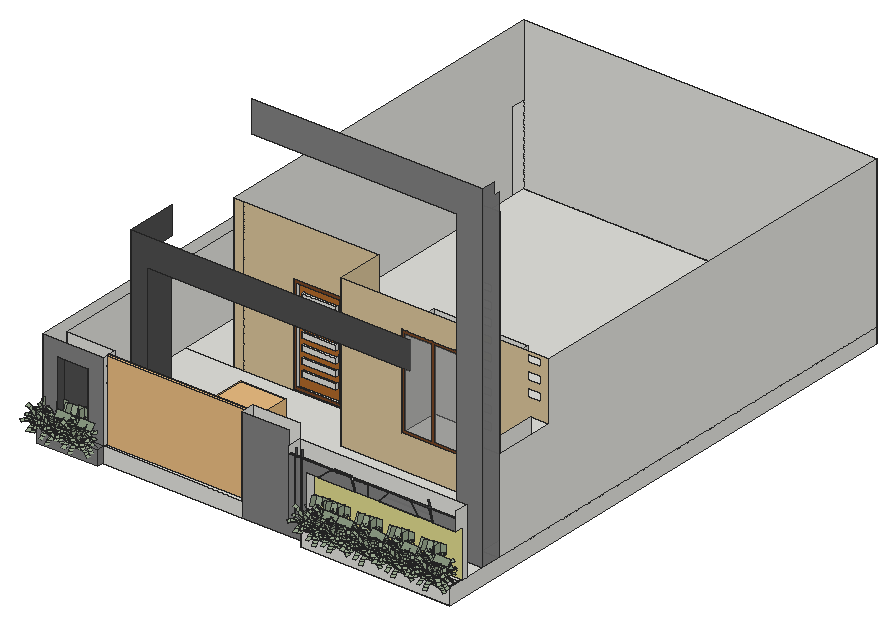
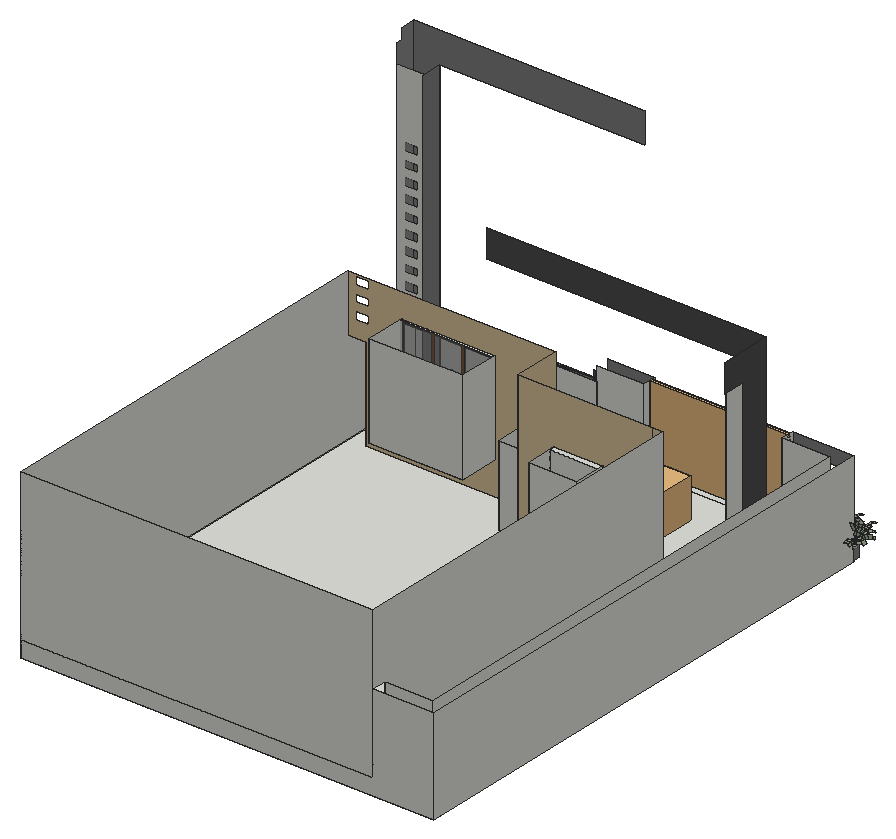
# SketchUp Ruby script. Lengths in inches.
U = 1.inch
M = Sketchup.active_model
def pt(a) = Geom::Point3d.new(a.map { |v| v * U })
def face(e, loops, mat)
  f = e.add_face(loops[0].map { |a| pt(a) })
  loops[1..].each { |l| e.add_face(l.map { |a| pt(a) }).erase! }
  f.material = f.back_material = mat if mat
  f
end
# faces: each face lists its corners as indices into pts; further lists are holes
def faces(e, pts, list, mat = nil) = list.each { |f| face(e, (f[0].is_a?(Array) ? f : [f]).map { |l| l.map { |i| pts[i] } }, mat) }
# xy, xz, yz: faces in a plane at the given z, y or x. An outline is a flat list of corners, or four numbers for a rectangle; further outlines are holes
def ring(l) = l.size == 4 ? [[l[0], l[1]], [l[2], l[1]], [l[2], l[3]], [l[0], l[3]]] : l.each_slice(2).to_a
def flat(e, list, mat, &to3) = list.each { |f| face(e, (f[0].is_a?(Array) ? f : [f]).map { |l| ring(l).map { |u, v| to3.(u, v) } }, mat) }
def xy(e, z, list, mat = nil) = flat(e, list, mat) { |x, y| [x, y, z] }
def xz(e, y, list, mat = nil) = flat(e, list, mat) { |x, z| [x, y, z] }
def yz(e, x, list, mat = nil) = flat(e, list, mat) { |y, z| [x, y, z] }
def lines(e, pts, list) = list.each { |a, b| e.add_line(pt(pts[a]), pt(pts[b])) }
# prism: a flat outline (further loops are holes) pulled along v
def prism(e, loops, v, mat = nil)
  f = face(e, loops, mat); d = Geom::Vector3d.new(v.map { |x| x * U })
  f.pushpull(f.normal.samedirection?(d) ? d.length : -d.length)
end
def box(e, o, s, mat = nil) = prism(e, [[o, [o[0] + s[0], o[1], o[2]], [o[0] + s[0], o[1] + s[1], o[2]], [o[0], o[1] + s[1], o[2]]]], [0, 0, s[2]], mat)
def at(x, y, z, deg = 0) = Geom::Transformation.translation(pt([x, y, z])) * Geom::Transformation.rotation(ORIGIN, Z_AXIS, deg.degrees)
def axes(o, x, y, z) = Geom::Transformation.new([*x, 0, *y, 0, *z, 0, *pt(o).to_a, 1])
def part(name) = M.definitions.add(name)
# library, detail: a bought-in or finely detailed component or shape, given as its bounding box
def library(name, o, s) = part(name).tap { |d| box(d.entities, o, s) }
def detail(e, o, s) = box(e.add_group.entities, o, s)
def put(e, d, t, mat = nil) = e.add_instance(d, t).tap { |i| i.material = mat if mat }
def group(e, t, mat = nil) = e.add_group.tap { |g| g.transformation = t; g.material = mat if mat }.entities
root = M.entities
M.materials.add("Generic").color = [129, 129, 129]
M.materials["Generic"].alpha = 0.97
M.materials.add("Generic\#1").color = [79, 79, 79]
M.materials.add("Generic\#3").color = [219, 197, 155]
M.materials.add("Generic\#5").color = [224, 219, 143]
M.materials.add("Generic\#6").color = [129, 129, 129]
M.materials.add("[Translucent Glass Gray]").color = [128, 128, 128]
M.materials["[Translucent Glass Gray]"].alpha = 0.28
M.materials.add("[Wood Bamboo]").color = [177, 105, 43]
M.materials.add("[Wood Board Cork]").color = [198, 185, 106]
M.materials.add("[Wood Veneer 01]").color = [120, 70, 37]
M.materials.add("hymenocallis littoralis").color = [156, 172, 146]
c1 = library("Group3\#1",[-238.15,54.18,0],[46.4,43.96,56.68])
c2 = part("Group\#856")
xy(c2.entities,7.38,[[0,0,5.5,15.91]],"hymenocallis littoralis")
p = [[5.5,28.78,0],[5.5,26.79,3.44],[0,26.79,3.44],[0,28.78,0],[0,23.75,6],[5.5,23.75,6],
  [0,15.91,7.38],[5.5,15.91,7.38]]
faces(c2.entities,p,[[0,1,2,3],[4,2,1,5],[6,4,5,7]],"hymenocallis littoralis")
c3 = part("Group\#854")
xy(c3.entities,7.38,[[0,0,5.5,15.91],[0,15.91,5.5,23.87]],"hymenocallis littoralis")
p = [[5.5,31.07,4.3],[5.5,27.74,6.47],[0,27.74,6.47],[0,31.07,4.3],[0,23.87,7.38],[5.5,23.87,7.38]]
faces(c3.entities,p,[[0,1,2,3],[4,2,1,5]],"hymenocallis littoralis")
c4 = part("Group\#857")
xy(c4.entities,7.38,[[0,0,5.6,15.91]],"hymenocallis littoralis")
p = [[5.6,28.78,0],[5.6,26.79,3.44],[0,26.79,3.44],[0,28.78,0],[0,23.75,6],[5.6,23.75,6],
  [0,15.91,7.38],[5.6,15.91,7.38]]
faces(c4.entities,p,[[0,1,2,3],[4,2,1,5],[6,4,5,7]],"hymenocallis littoralis")
c5 = part("Group\#855")
put(c5.entities,c3,axes([6.09,8.57,-0.52],[0.446,0.85617,0.26089],[-0.18444,-0.19731,0.96283],[0.87582,-0.47754,0.0699]))
put(c5.entities,c3,axes([6.29,7.28,-1.71],[0.37058,0.92707,-0.05667],[-0.32382,0.19004,0.99128],[0.87712,-0.32925,0.34964]))
put(c5.entities,c3,axes([11.04,16.14,-0.7],[1,0,0],[0,0.16628,1.02662],[0,-1.18456,0.19186]))
c6 = part("Group\#860")
put(c6.entities,c2,axes([24.57,32.05,-1.76],[0.9552,-0.22102,-0.19681],[0.4036,0.95545,0.88585],[-0.00568,-0.67859,0.7345]))
put(c6.entities,c2,axes([23.95,29.24,-2.4],[0,1,0],[-0.76041,0,0.64945],[0.64945,0,0.76041]))
put(c6.entities,c2,axes([24.22,24.72,-0.48],[-0.70711,0.70711,0],[-0.32757,-0.32757,0.80237],[0.61237,0.61237,0.5]))
put(c6.entities,c3,axes([20.66,37.22,-0.63],[1.12361,0.03262,0.39091],[-0.43499,0.29739,0.78777],[0.09852,-1.27434,0.37535]))
put(c6.entities,c2,axes([28.75,24.45,-2.4],[-1,0,0],[0,-0.76041,0.64945],[0,0.64945,0.76041]))
put(c6.entities,c4,axes([30.4,30.98,-3.7],[0.65676,-0.72002,0.22414],[0.55667,0.66341,0.5],[-0.50871,-0.20361,0.83652]))
put(c6.entities,c4,axes([32.41,29.61,-3.7],[0.04029,-0.97372,0.22414],[0.85287,0.15038,0.5],[-0.52057,0.17102,0.83652]))
put(c6.entities,c2,axes([31.89,25.85,-1.76],[-0.92056,0.33739,-0.19681],[-0.5186,-0.89824,0.88585],[0.08952,0.67268,0.7345]))
put(c6.entities,c2,axes([25.55,34.78,-0.48],[0.86603,0.5,0],[-0.25,0.43301,0.86603],[0.43301,-0.75,0.5]))
put(c6.entities,c4,axes([20.4,16.9375,-8.07],[-0.70711,0.70711,0],[-0.35754,-0.35754,0.65422],[1.3987,1.3987,1.52882]))
put(c6.entities,c2,axes([32.86,34.14,-0.48],[0.76604,-0.64279,0],[0.32139,0.38302,0.86603],[-0.55667,-0.66341,0.5]))
put(c6.entities,c2,axes([27.15,34.7,-0.1],[0.82472,-0.17528,-0.53769],[0.53769,0.53769,0.64945],[0.17528,-0.82472,0.53769]))
put(c6.entities,c2,axes([33.58,28.77,-2.4],[0,-1,0],[0.76041,0,0.64945],[-0.64945,0,0.76041]))
put(c6.entities,c2,axes([26.43,23.87,-2.81],[-0.75126,0.04415,0.65853],[0.53769,-0.53769,0.64945],[0.38276,0.84199,0.3802]))
put(c6.entities,c2,axes([28.78,23.98,-2.4],[-1,0,0],[0,-0.76041,0.64945],[0,0.64945,0.76041]))
put(c6.entities,c2,axes([25.39,25.38,-2.4],[-0.70711,0.70711,0],[-0.53769,-0.53769,0.64945],[0.45923,0.45923,0.76041]))
put(c6.entities,c2,axes([27.32,21.63,-0.1],[-0.45923,0.70711,-0.53769],[-0.76041,0,0.64945],[0.45923,0.70711,0.53769]))
put(c6.entities,c2,axes([25.17,27.625,-1.76],[0.56416,0.80187,-0.19681],[-0.66673,0.66673,0.80532],[0.62659,-0.26057,0.7345]))
put(c6.entities,c4,axes([27.59,27.04,-3.96],[-0.8993,-0.06127,0.43301],[0.2962,-0.8138,0.5],[0.32175,0.57791,0.75]))
put(c6.entities,c4,axes([26.98,24.5,-3.18],[-0.5,0.86603,0],[-0.75,-0.43301,0.5],[0.43301,0.25,0.86603]))
put(c6.entities,c4,axes([24.55,27.74,-3.7],[0.29517,0.92878,0.22414],[-0.85287,0.15038,0.5],[0.43068,-0.33875,0.83652]))
put(c6.entities,c4,axes([24.26,29.8,-3.18],[0.76604,0.64279,0],[-0.47317,0.5639,0.425],[0.32139,-0.38302,0.86603]))
put(c6.entities,c4,axes([25.98,32.46,-3.18],[1,0,0],[0,0.86603,0.5],[0,-0.5,0.86603]))
put(c6.entities,c2,axes([28.78,33.57,-2.4],[1,0,0],[0,0.76041,0.64945],[0,-0.64945,0.76041]))
put(c6.entities,c5,at(14.99,21.38,2.5))
put(c6.entities,c3,axes([34.63,26.34,-1.46],[-0.70089,-0.70877,0.07994],[0.4756,-0.38088,0.79293],[-0.53156,0.59378,0.60405]))
put(c6.entities,c3,axes([28.14,16.92,1.8125],[-1.19719,0.6912,0],[-0.09607,-0.16641,0.94244],[0.68444,1.18549,0.17613]))
put(c6.entities,c3,axes([31.5625,35.84,0.97],[0.66765,-1.1564,0.35779],[0.04445,0.30732,0.91033],[-1.20828,-0.64496,0.17012]))
put(c6.entities,c3,axes([38.94,22.51,0.89],[-0.97932,-0.67164,-0.05202],[0.27787,-0.41401,0.90999],[-0.85985,0.93577,0.32097]))
put(c6.entities,c3,axes([38.44,21.09,1.98],[-1.02864,-0.54856,0.2395],[0.33481,0.06999,0.88388],[-0.77261,1.08328,0.06417]))
put(c6.entities,c4,axes([35.02,30.51,-1.3],[-0.17365,-0.98481,0],[0.60224,-0.10619,0.79122],[-0.7792,0.13739,0.61153]))
put(c6.entities,c4,axes([29.41,22.33,-1.3],[-0.93969,0.34202,0],[-0.20915,-0.57465,0.79122],[0.27061,0.74351,0.61153]))
put(c6.entities,c3,axes([19.64,36,-1.62],[1.18194,0.09546,0.08234],[-0.14377,0.68823,0.76313],[0.21457,-1.1326,0.62386]))
put(c6.entities,c4,axes([24.25,24.14,-1.3],[-0.34202,0.93969,0],[-0.57465,-0.20915,0.79122],[0.74351,0.27061,0.61153]))
put(c6.entities,c4,axes([25.98,34.61,-1.3],[1,0,0],[0,0.61153,0.79122],[0,-0.79122,0.61153]))
put(c6.entities,c4,axes([31.16,34.41,-1.64],[0.56518,-0.80224,-0.19234],[0.73413,0.34233,0.72935],[-0.47639,-0.50772,0.71782]))
put(c6.entities,c4,axes([40.52,26.84,-5.82],[-0.42262,-0.90631,0],[0.48019,-0.22391,0.68552],[-1.43418,0.66877,1.22305]))
put(c6.entities,c2,axes([29.86,38.42,-1.01],[0.89064,-0.37013,0.26413],[-0.03924,0.63286,1.01918],[-0.45353,-0.76487,0.45748]))
put(c6.entities,c2,axes([29.34,22.4,-0.48],[-0.99619,-0.08716,0],[0.04358,-0.4981,0.86603],[-0.07548,0.86273,0.5]))
c7 = part("Group\#858")
xz(c7.entities,10.07,[[9.07,0,10.07,31.01],[0,31.01,0,45.12,20.13,45.12,20.13,31.01,10.07,31.01,10.07,32.58,9.07,32.58,9.07,31.01]],"hymenocallis littoralis")
yz(c7.entities,10.07,[[0,31.01,20.13,45.12]],"hymenocallis littoralis")
p = [[9.57,9.2,0],[10.07,10.07,0],[10.07,10.07,31.01],[10.07,10.07,32.58],[9.57,9.2,32.58]]
faces(c7.entities,p,[[0,1,2,3,4]],"hymenocallis littoralis")
c8 = part("cây lá nắng")
put(c8.entities,c6,axes([49.26,-2.75,0],[0.63109,0.63109,0],[-0.63109,0.63109,0],[0,0,0.935]))
g1 = group(c8.entities,at(26.6,-8.68,0))
put(g1,c2,axes([-4.72,35.73,-1.65],[0.74231,0.46334,-0.18402],[-0.34827,0.85768,0.82827],[0.42467,-0.43184,0.68675]))
put(g1,c2,axes([-3.34,33.57,-2.24],[-0.63109,0.63109,0],[-0.47989,-0.47989,0.60723],[0.40986,0.40986,0.71098]))
put(g1,c2,axes([-0.3125,30.89,-0.45],[-0.8925,0,0],[0,-0.41345,0.75022],[0,0.77293,0.4675]))
put(g1,c3,axes([-10.79,39.66,-0.59],[0.68852,0.72969,0.3655],[-0.4622,-0.08684,0.73657],[0.86641,-0.74205,0.35095]))
put(g1,c2,axes([2.71,33.57,-2.24],[-0.63109,-0.63109,0],[0.47989,-0.47989,0.60723],[-0.40986,0.40986,0.71098]))
put(g1,c4,axes([-0.37,38.74,-3.46],[0.86887,-0.03992,0.20957],[-0.06737,0.76999,0.4675],[-0.19255,-0.44954,0.78214]))
put(g1,c4,axes([1.76,39.14,-3.46],[0.63993,-0.58908,0.20957],[0.44333,0.63315,0.4675],[-0.43646,-0.2206,0.78214]))
put(g1,c2,axes([3.81,36.4375,-1.65],[-0.79389,-0.36803,-0.18402],[0.23959,-0.89415,0.82827],[-0.36803,0.48102,0.68675]))
put(g1,c2,axes([-5.83,38.07,-0.45],[0.231,0.86209,0],[-0.43104,0.1155,0.80973],[0.74659,-0.20005,0.4675]))
put(g1,c4,axes([2.18,23.5625,-7.55],[-0.8925,0,0],[0,-0.45128,0.6117],[0,1.76542,1.42944]))
put(g1,c2,axes([-0.8125,42.28,-0.45],[0.8891,0.07779,0],[-0.03889,0.44455,0.80973],[0.06737,-0.76999,0.4675]))
put(g1,c2,axes([-4.76,39.03,-0.09],[0.63109,0.40986,-0.50274],[0,0.67866,0.60723],[0.63109,-0.40986,0.50274]))
put(g1,c2,axes([3.03,39.35,-2.24],[0.63109,-0.63109,0],[0.47989,0.47989,0.60723],[-0.40986,-0.40986,0.71098]))
put(g1,c2,axes([1.61,31.74,-2.625],[-0.50198,-0.44625,0.61573],[0.67866,0,0.60723],[-0.28982,0.77293,0.35549]))
put(g1,c2,axes([3.03,33.3,-2.24],[-0.63109,-0.63109,0],[0.47989,-0.47989,0.60723],[-0.40986,0.40986,0.71098]))
put(g1,c2,axes([0.01,32.04,-2.24],[-0.8925,0,0],[0,-0.67866,0.60723],[0,0.57963,0.71098]))
put(g1,c2,axes([3.59,30.89,-0.09],[-0.73607,0.15643,-0.50274],[-0.47989,-0.47989,0.60723],[-0.15643,0.73607,0.50274]))
put(g1,c2,axes([-1.55,33.32,-1.65],[-0.15002,0.86209,-0.18402],[-0.84154,0,0.75297],[0.55988,0.231,0.68675]))
put(g1,c4,axes([0.35,34.48,-3.71],[-0.52887,-0.60621,0.40487],[0.70051,-0.32665,0.4675],[-0.16166,0.56777,0.70125]))
put(g1,c4,axes([2.61,39.13,-1.74],[-0.86209,0.231,0],[-0.23031,-0.85954,0.15531],[0.03162,0.11799,0.91645]))
put(g1,c4,axes([-2.02,33,-3.46],[-0.39986,0.77243,0.20957],[-0.63315,-0.44333,0.4675],[0.48558,0.05802,0.78214]))
put(g1,c4,axes([-3.49,34.12,-2.97],[0.07779,0.8891,0],[-0.65449,0.05726,0.39737],[0.44455,-0.03889,0.80973]))
put(g1,c4,axes([-4.09,36.88,-2.97],[0.63109,0.63109,0],[-0.54654,0.54654,0.4675],[0.31555,-0.31555,0.80973]))
put(g1,c2,axes([-3.02,39.35,-2.24],[0.63109,0.63109,0],[-0.47989,0.47989,0.60723],[0.40986,-0.40986,0.71098]))
put(g1,c5,axes([-4.03,22.95,2.33],[0.63109,0.63109,0],[-0.63109,0.63109,0],[0,0,0.935]))
put(g1,c3,axes([5.24,38.48,-1.37],[0.00497,-0.88963,0.07474],[0.54052,0.05978,0.74139],[-0.71019,0.03927,0.56479]))
put(g1,c3,axes([7.08,28.4375,1.7],[-1.19175,-0.31933,0],[0.04439,-0.16565,0.88118],[-0.31621,1.1801,0.16468]))
put(g1,c3,axes([-2.7,42.54,0.91],[1.15114,-0.30845,0.33454],[-0.1659,0.22199,0.85115],[-0.3555,-1.16957,0.15907]))
put(g1,c3,axes([10.37,38.78,0.83],[-0.19417,-1.04191,-0.04864],[0.43664,-0.08592,0.85084],[-1.1332,0.04791,0.30011]))
put(g1,c3,axes([10.95,37.5625,1.85],[-0.30298,-0.99536,0.22393],[0.16713,0.25547,0.82643],[-1.17124,0.19607,0.06]))
put(g1,c4,axes([2.84,41.36,-1.22],[0.51192,-0.73109,0],[0.44708,0.31305,0.73979],[-0.57846,-0.40504,0.57178]))
put(g1,c4,axes([4.47,32.65,-1.22],[-0.80888,-0.37719,0],[0.23066,-0.49465,0.73979],[-0.29844,0.64,0.57178]))
put(g1,c3,axes([-10.32,35.12,-1.51],[0.68567,0.80616,0.07699],[-0.52507,0.3436,0.71352],[0.85019,-0.57936,0.58331]))
put(g1,c4,axes([0.07,30.54,-1.22],[-0.80888,0.37719,0],[-0.23066,-0.49465,0.73979],[0.29844,0.64,0.57178]))
put(g1,c4,axes([-5.45,38.24,-1.22],[0.63109,0.63109,0],[-0.38593,0.38593,0.73979],[0.49934,-0.49934,0.57178]))
put(g1,c4,axes([-2.05,41.38,-1.53],[0.86296,-0.14961,-0.17984],[0.24726,0.67935,0.68194],[0.01977,-0.62107,0.67116]))
put(g1,c4,axes([8.63,42.51,-5.4375],[0.30525,-0.83868,0],[0.44435,0.16173,0.64096],[-1.32716,-0.48305,1.14356]))
put(g1,c2,axes([-5.4,43.09,-0.94],[0.79566,0.32849,0.24696],[-0.42416,0.37462,0.95293],[0.19648,-0.76892,0.42774]))
put(g1,c2,axes([4.38,32.65,-0.45],[-0.57369,-0.68369,0],[0.34185,-0.28684,0.80973],[-0.5921,0.49683,0.4675]))
put(g1,c4,axes([-2,33.84,-0.15],[-0.24601,0.85793,0],[-0.85539,-0.24528,0.15531],[0.11742,0.03367,0.91645]))
put(g1,c4,axes([0.17,30.83,-4.47],[-0.24601,0.85793,0],[-0.85539,-0.24528,0.15531],[0.11742,0.03367,0.91645]))
put(g1,c4,axes([-1.97,32.18,-4.47],[0.58524,0.67383,0],[-0.67184,0.58351,0.15531],[0.09222,-0.0801,0.91645]))
put(g1,c4,axes([-2,34.71,-4.47],[0.88392,-0.12346,0],[0.12309,0.88131,0.15531],[-0.0169,-0.12098,0.91645]))
put(g1,c4,axes([0.11,36.12,-4.47],[0.37822,-0.8084,0],[0.80601,0.37711,0.15531],[-0.11064,-0.05177,0.91645]))
put(c8.entities,c7,axes([29.71,14.29,6.94],[0.425,0.73612,0],[-0.6771,0.39092,-0.33349],[-0.26859,0.15507,0.72712]))
put(c8.entities,c7,axes([42.0625,26.12,6.94],[0.85,0,0],[0,0.78185,-0.33349],[0,0.33349,0.78185]))
put(c8.entities,c6,axes([7.3125,23.0625,0],[0.8925,0,0],[0,0.8925,0],[0,0,0.935]))
put(c8.entities,c7,axes([24.4375,40.23,2.05],[0.85,0,0],[0,0.85,0],[0,0,0.85]))
c9 = part("Planting+101")
put(c9.entities,c8,axes([21.34,32.96,-4.59],[0,-0.71,0],[-0.71,0,0],[0,0,0.71]))
c10 = library("Group\#1",[0,0,0],[141.125,3.24,81.5])
c11 = library("Group\#6",[0,0,0],[4.375,32.17,82.28])
c12 = part("Group\#5")
xy(c12.entities,0,[[0,2.125,49.6875,7.875]])
xy(c12.entities,2.71,[[2.71,2.125,46.98,4.875]])
xy(c12.entities,13.9,[[8.49,2.125,42.99,4.875]])
xy(c12.entities,19.09,[[8.49,2.125,42.99,4.875]])
xy(c12.entities,25.71,[[8.49,2.125,42.99,4.875]])
xy(c12.entities,30.9,[[8.49,2.125,42.99,4.875]])
xy(c12.entities,37.52,[[8.49,2.125,42.99,4.875]])
xy(c12.entities,42.71,[[8.49,2.125,42.99,4.875]])
xy(c12.entities,49.34,[[8.49,2.125,42.99,4.875]])
xy(c12.entities,54.52,[[8.49,2.125,42.99,4.875]])
xy(c12.entities,61.15,[[8.49,2.125,42.99,4.875]])
xy(c12.entities,66.34,[[8.49,2.125,42.99,4.875]])
xy(c12.entities,72.96,[[8.49,2.125,42.99,4.875]])
xy(c12.entities,78.15,[[8.49,2.125,42.99,4.875]])
xy(c12.entities,84.77,[[8.49,2.125,42.99,4.875]])
xy(c12.entities,89.96,[[8.49,2.125,42.99,4.875]])
xy(c12.entities,97.73,[[2.71,2.125,46.98,4.875]])
xy(c12.entities,100.4375,[[0,2.125,49.6875,7.875]])
xz(c12.entities,0,[[48.27,47.74,48.43,47.76,48.58,47.82,48.71,47.92,48.8125,48.05,48.875,48.2,48.89,48.36,48.875,48.52,48.8125,48.67,48.71,48.8,48.58,48.9,48.43,48.97,48.27,48.99,48.11,48.97,47.96,48.9,47.83,48.8,47.73,48.67,47.67,48.52,47.64,48.36,47.67,48.2,47.73,48.05,47.83,47.92,47.96,47.82,48.11,47.76]])
xz(c12.entities,2.125,[[8.49,13.9,42.99,19.09],[8.49,25.71,42.99,30.9],[8.49,37.52,42.99,42.71],[48.27,47.74,48.11,47.76,47.96,47.82,47.83,47.92,47.73,48.05,47.67,48.2,47.64,48.36,47.67,48.52,47.73,48.67,47.83,48.8,47.96,48.9,48.11,48.97,48.27,48.99,48.43,48.97,48.58,48.9,48.71,48.8,48.8125,48.67,48.875,48.52,48.89,48.36,48.875,48.2,48.8125,48.05,48.71,47.92,48.58,47.82,48.43,47.76],[8.49,49.34,42.99,54.52],
  [8.49,61.15,42.99,66.34],[8.49,72.96,42.99,78.15],[8.49,84.77,42.99,89.96]])
xz(c12.entities,2.125,[[[0,0,49.6875,100.4375],[2.71,2.71,46.98,97.73],[48.27,47.74,48.11,47.76,47.96,47.82,47.83,47.92,47.73,48.05,47.67,48.2,47.64,48.36,47.67,48.52,47.73,48.67,47.83,48.8,47.96,48.9,48.11,48.97,48.27,48.99,48.43,48.97,48.58,48.9,48.71,48.8,48.8125,48.67,48.875,48.52,48.89,48.36,48.875,48.2,48.8125,48.05,48.71,47.92,48.58,47.82,48.43,47.76]]],"[Wood Veneer 01]")
xz(c12.entities,4.875,[[[2.71,2.71,46.98,97.73],[8.49,84.77,42.99,89.96],[8.49,72.96,42.99,78.15],[8.49,61.15,42.99,66.34],[8.49,49.34,42.99,54.52],[8.49,37.52,42.99,42.71],[8.49,25.71,42.99,30.9],[8.49,13.9,42.99,19.09]]],"[Wood Bamboo]")
xz(c12.entities,7.875,[[0,0,49.6875,100.4375]])
yz(c12.entities,0,[[2.125,0,7.875,100.4375]])
yz(c12.entities,2.71,[[2.125,2.71,4.875,97.73]])
yz(c12.entities,8.49,[[2.125,13.9,4.875,19.09],[2.125,25.71,4.875,30.9],[2.125,37.52,4.875,42.71],[2.125,49.34,4.875,54.52],[2.125,61.15,4.875,66.34],
  [2.125,72.96,4.875,78.15],[2.125,84.77,4.875,89.96]])
yz(c12.entities,42.99,[[2.125,13.9,4.875,19.09],[2.125,25.71,4.875,30.9],[2.125,37.52,4.875,42.71],[2.125,49.34,4.875,54.52],[2.125,61.15,4.875,66.34],
  [2.125,72.96,4.875,78.15],[2.125,84.77,4.875,89.96]])
yz(c12.entities,46.98,[[2.125,2.71,4.875,97.73]])
yz(c12.entities,49.6875,[[2.125,0,7.875,100.4375]])
p = [[48.11,2.125,47.76],[48.27,2.125,47.74],[48.27,0,47.74],[48.11,0,47.76],[48.43,2.125,47.76],[48.43,0,47.76],
  [47.83,2.125,47.92],[47.96,2.125,47.82],[47.96,0,47.82],[47.83,0,47.92],[48.58,2.125,47.82],[48.58,0,47.82],
  [48.71,2.125,47.92],[48.71,0,47.92],[47.73,2.125,48.05],[47.73,0,48.05],[48.8125,2.125,48.05],[48.8125,0,48.05],
  [47.67,2.125,48.2],[47.67,0,48.2],[48.875,2.125,48.2],[48.875,0,48.2],[47.64,2.125,48.36],[47.64,0,48.36],
  [48.89,2.125,48.36],[48.89,0,48.36],[47.67,2.125,48.52],[47.67,0,48.52],[48.875,2.125,48.52],[48.875,0,48.52],
  [47.73,2.125,48.67],[47.73,0,48.67],[48.8125,2.125,48.67],[48.8125,0,48.67],[47.83,2.125,48.8],[47.83,0,48.8],
  [48.71,2.125,48.8],[48.71,0,48.8],[47.96,2.125,48.9],[47.96,0,48.9],[48.58,2.125,48.9],[48.58,0,48.9],
  [48.11,2.125,48.97],[48.11,0,48.97],[48.43,2.125,48.97],[48.43,0,48.97],[48.27,2.125,48.99],[48.27,0,48.99],
  [48.27,2.125,48.36],[48.27,0,48.36]]
faces(c12.entities,p,[[0,1,2,3],[1,4,5,2],[6,7,8,9],[7,0,3,8],[4,10,11,5],[10,12,13,11],[14,6,9,15],[12,16,17,13],
  [18,14,15,19],[16,20,21,17],[22,18,19,23],[20,24,25,21],[26,22,23,27],[24,28,29,25],[30,26,27,31],[28,32,33,29],
  [34,30,31,35],[32,36,37,33],[38,34,35,39],[36,40,41,37],[42,38,39,43],[40,44,45,41],[46,42,43,47],[44,46,47,45]])
lines(c12.entities,p,[[48,49]])
xy(root,-26.1875,[[283.58,20.95,283.58,28.58,13.36,28.58,13.36,565.96,435.86,565.96,435.86,20.95]])
xy(root,-26.1875,[[13.36,20.95,75.86,28.58]],"Generic")
xy(root,-20.0625,[[285.53,22.47,433.91,35.38]])
xy(root,-10.3125,[[[283.58,20.95,435.86,37.33],[285.53,22.47,433.91,35.38]],[75.86,28.58,216.99,42.52],[264.86,28.58,264.86,42.52,435.86,42.52,435.86,37.33,283.58,37.33,283.58,28.58,278.21,28.58,278.21,29.64,277.21,29.64,277.21,28.58,272.42,28.58,272.42,29.64,271.42,29.64,271.42,28.58],[271.42,28.58,272.42,29.64],[277.21,28.58,278.21,29.64],
  [[26.8,42.52,435.86,42.52,435.86,62.71,409.3,62.71,409.3,84.21,418.23,84.21,418.23,146.83,223.67,146.83,223.67,155.49,249.48,155.49,249.48,187.55,223.67,187.55,223.67,194.96,26.8,194.96],[75.86,62.71,93.35,92.14]],[418.23,84.21,435.86,84.21,435.86,565.96,75.86,565.96,75.86,194.96,223.67,194.96,223.67,187.55,249.48,187.55,249.48,155.49,223.67,155.49,223.67,146.83,418.23,146.83],[26.8,194.96,75.86,550.64]])
xy(root,-10.23,[[29.32,28.58,59.9,36.21]],"Generic\#1")
xy(root,-8.96,[[137.0625,194.96,186.75,227.77]])
xy(root,23.6,[[286.0625,146.83,381.5625,188.08]])
xy(root,38.09,[[283.58,28.58,283.58,37.33,435.86,37.33,435.86,28.58,412.22,28.58,412.22,29.27,411.22,29.27,411.22,28.58,397.92,28.58,397.92,29.27,396.92,29.27,396.92,28.58,357.98,28.58,357.98,28.77,356.98,28.77,356.98,28.58,346.31,28.58,346.31,29.02,345.31,29.02,345.31,28.58,333.23,28.58,333.23,29.02,332.23,29.02,332.23,28.58,295.29,28.58,295.29,29.02,294.29,29.02,294.29,28.58]])
xy(root,49.4375,[[329.86,28.58,345.31,28.77],[346.31,28.58,366.89,28.77],[409.57,28.58,435.86,29.27],[309.31,29.27,328.86,30.14]])
xy(root,49.4375,[[264.86,28.58,271.42,29.64],[272.42,28.58,277.21,29.64],[278.21,28.58,308.31,28.58,308.31,29.02,309.31,29.02,309.31,29.64,278.21,29.64],[309.31,28.58,328.86,29.27],[367.89,28.58,389.59,28.58,389.59,29.27,328.86,29.27,328.86,29.02,329.86,29.02,329.86,28.77,345.31,28.77,345.31,29.02,346.31,29.02,346.31,28.77,367.89,28.77],
  [390.59,28.58,408.57,29.27]],"Generic\#1")
xz(root,20.95,[[283.58,-26.1875,435.86,-10.3125]])
xz(root,20.95,[[13.36,-26.1875,75.86,-26.1875,75.86,-10.3125,59.9,-10.23,29.32,-10.23,13.36,-10.14]],"Generic")
xz(root,22.47,[[285.53,-20.0625,433.91,-10.3125]])
xz(root,28.58,[[75.86,-26.1875,216.99,-10.3125]])
xz(root,28.58,[[13.36,-26.1875,13.36,-10.14,29.32,-10.23,59.9,-10.23,75.86,-10.3125,75.86,-26.1875],[264.86,-10.3125,271.42,49.4375],[272.42,-10.3125,277.21,49.4375],[357.98,38.09,396.92,38.09,389.59,49.4375,367.89,49.4375],[397.92,38.09,411.22,38.09,408.57,49.4375,390.59,49.4375]],"Generic")
xz(root,28.58,[[216.99,-26.1875,283.58,-26.1875,283.58,-10.3125,264.86,-10.3125,264.86,71.1875,216.99,71.1875],[75.86,-10.3125,75.86,71.1875,13.36,71.1875,13.36,-10.14,29.32,-10.23,29.32,55.23,59.9,55.23,59.9,-10.23],[278.21,-10.3125,283.58,-10.3125,283.58,38.09,294.29,38.09,308.31,49.4375,278.21,49.4375],[295.29,38.09,332.23,38.09,328.86,49.4375,309.31,49.4375],[333.23,38.09,345.31,38.09,345.31,49.4375,329.86,49.4375],
  [346.31,38.09,356.98,38.09,366.89,49.4375,346.31,49.4375],[412.22,38.09,435.86,38.09,435.86,49.4375,409.57,49.4375]],"Generic\#6")
xz(root,28.77,[[356.98,38.09,357.98,38.09,367.89,49.4375,366.89,49.4375]],"Generic\#1")
xz(root,29.02,[[294.29,38.09,295.29,38.09,309.31,49.4375,308.31,49.4375],[332.23,38.09,333.23,38.09,329.86,49.4375,328.86,49.4375],[345.31,38.09,346.31,49.4375]],"Generic\#1")
xz(root,29.27,[[396.92,38.09,397.92,38.09,390.59,49.4375,408.57,49.4375,411.22,38.09,412.22,38.09,409.57,49.4375,435.86,49.4375,435.86,50.4375,409.34,50.4375,407.85,56.8125,406.85,56.8125,408.34,50.4375,310.55,50.4375,309.31,49.4375,389.59,49.4375]],"Generic\#1")
xz(root,29.64,[[271.42,-10.3125,272.42,56.8125],[277.21,-10.3125,278.21,56.8125],[264.86,49.4375,271.42,50.4375],[272.42,49.4375,277.21,50.4375],[278.21,49.4375,309.31,49.4375,310.55,50.4375,278.21,50.4375]],"Generic\#1")
xz(root,30.14,[[309.31,49.4375,310.55,50.4375,328.5625,50.4375,328.86,49.4375]])
xz(root,35.38,[[285.53,-20.0625,433.91,-10.3125]])
xz(root,36.21,[[29.32,-10.23,59.9,55.23]],"Generic\#1")
xz(root,37.33,[[283.58,-10.3125,435.86,38.09]],"Generic\#5")
xz(root,42.52,[[26.8,-10.3125,75.86,71.1875],[216.99,-10.3125,264.86,71.1875],[264.86,-10.3125,435.86,56.8125]])
xz(root,62.71,[[75.86,-10.3125,93.35,-10.3125,93.35,144,361.3125,144,361.3125,172.625,75.86,172.625]],"Generic\#1")
xz(root,62.71,[[409.3,-10.3125,435.86,-10.3125,435.86,336.625,200.23,336.625,200.23,304.8125,409.3,304.8125]],"Generic\#6")
xz(root,84.21,[[[409.3,-10.3125,409.3,306.4375,435.86,306.4375,435.86,85.23,418.23,85.23,418.23,-10.3125],[415.03,102.26,427.87,110.19],[415.03,118.13,427.87,126.07],[415.03,134.01,427.87,141.94],[415.03,149.88,427.87,157.82],[415.03,165.76,427.87,173.69],[415.03,181.63,427.87,189.57],[415.03,197.51,427.87,205.44],[415.03,213.38,427.87,221.32],[415.03,229.26,427.87,237.19]]])
xz(root,92.14,[[75.86,-10.3125,93.35,144]])
xz(root,146.83,[[[223.67,-10.3125,418.23,-10.3125,418.23,85.23,435.86,85.23,435.86,144,223.67,144],[286.0625,23.6,381.5625,119.1],[415.03,102.26,427.87,110.19],[415.03,118.13,427.87,126.07],[415.03,134.01,427.87,141.94]]],"Generic\#3")
xz(root,188.08,[[286.0625,23.6,381.5625,119.1]])
xz(root,194.96,[[75.86,-10.3125,86.05,144],[[86.05,-10.3125,223.67,144],[137.0625,-8.96,186.75,91.48]]],"Generic\#3")
xz(root,227.77,[[137.0625,-8.96,186.75,91.48]])
xz(root,550.64,[[26.8,-10.3125,75.86,71.1875]])
xz(root,565.96,[[13.36,-26.1875,13.36,71.1875,75.86,71.1875,75.86,-10.3125,435.86,-10.3125,435.86,-26.1875],[75.86,-10.3125,435.86,144]])
yz(root,13.36,[[28.58,-26.1875,565.96,71.1875]])
yz(root,13.36,[[20.95,-26.1875,28.58,-10.14]],"Generic")
yz(root,26.8,[[42.52,-10.3125,550.64,71.1875]])
yz(root,29.32,[[28.58,-10.23,36.21,55.23]],"Generic\#1")
yz(root,59.9,[[28.58,-10.23,36.21,55.23]],"Generic\#1")
yz(root,75.86,[[28.58,-10.3125,42.52,71.1875],[194.96,-10.3125,194.96,144,565.96,144,565.96,71.1875,550.64,71.1875,550.64,-10.3125]])
yz(root,75.86,[[20.95,-26.1875,28.58,-10.3125]],"Generic")
yz(root,75.86,[[62.71,-10.3125,62.71,172.625,115.77,172.625,115.77,144,92.14,144,92.14,-10.3125]],"Generic\#1")
yz(root,93.35,[[62.71,-10.3125,92.14,144]],"Generic\#1")
yz(root,137.0625,[[194.96,-8.96,227.77,91.48]])
yz(root,186.75,[[194.96,-8.96,227.77,91.48]])
yz(root,216.99,[[28.58,-10.3125,42.52,71.1875]])
yz(root,223.67,[[146.83,-10.3125,146.83,144,194.96,144,194.96,-10.3125,187.55,-10.3125,187.66,71.97,155.6,71.97,155.49,-10.3125]],"Generic\#3")
yz(root,249.48,[[155.49,-10.3125,155.6,71.97,187.66,71.97,187.55,-10.3125]])
yz(root,264.86,[[28.58,-10.3125,42.52,-10.3125,42.52,56.8125,28.58,56.8125,28.58,50.4375,29.64,50.4375,29.64,49.4375,28.58,49.4375],[28.58,49.4375,29.64,50.4375]])
yz(root,271.42,[[28.58,-10.3125,29.64,49.4375]],"Generic\#1")
yz(root,272.42,[[28.58,-10.3125,29.64,49.4375]],"Generic\#1")
yz(root,277.21,[[28.58,-10.3125,29.64,49.4375]],"Generic\#1")
yz(root,278.21,[[28.58,-10.3125,29.64,49.4375]],"Generic\#1")
yz(root,283.58,[[20.95,-26.1875,28.58,-10.3125],[28.58,-10.3125,37.33,38.09]])
yz(root,285.53,[[22.47,-20.0625,28.58,-10.3125],[28.58,-20.0625,35.38,-10.3125]])
yz(root,286.0625,[[146.83,23.6,188.08,119.1]])
yz(root,345.31,[[28.58,38.09,29.02,49.4375]],"Generic\#1")
yz(root,346.31,[[28.58,38.09,29.02,49.4375]],"Generic\#1")
yz(root,381.5625,[[146.83,23.6,188.08,119.1]])
yz(root,409.3,[[62.71,-10.3125,84.21,304.8125]],"Generic")
yz(root,418.23,[[84.21,-10.3125,146.83,85.23]])
yz(root,433.91,[[22.47,-20.0625,35.38,-10.3125]])
yz(root,435.86,[[20.95,-26.1875,565.96,-10.3125],[37.33,-10.3125,42.52,-10.3125,42.52,56.8125,28.58,56.8125,28.58,50.4375,29.27,50.4375,29.27,49.4375,28.58,49.4375,28.58,38.09,37.33,38.09],[84.21,-10.3125,565.96,-10.3125,565.96,144,146.83,144,146.83,85.23,84.21,85.23]])
yz(root,435.86,[[62.71,-10.3125,84.21,-10.3125,84.21,324.875,77.89,324.875,77.89,336.625,62.71,336.625]],"Generic")
p = [[223.67,155.49,-10.3125],[223.67,155.6,71.97],[249.48,155.6,71.97],[249.48,155.49,-10.3125],[223.67,187.66,71.97],[223.67,187.55,-10.3125],
  [249.48,187.55,-10.3125],[249.48,187.66,71.97],[308.31,28.58,49.4375],[294.29,28.58,38.09],[294.29,29.02,38.09],[308.31,29.02,49.4375],
  [295.29,28.58,38.09],[309.31,28.58,49.4375],[309.31,29.02,49.4375],[295.29,29.02,38.09],[328.86,28.58,49.4375],[332.23,28.58,38.09],
  [332.23,29.02,38.09],[328.86,29.02,49.4375],[333.23,28.58,38.09],[329.86,28.58,49.4375],[329.86,28.77,49.4375],[329.86,29.02,49.4375],
  [333.23,29.02,38.09],[366.89,28.58,49.4375],[356.98,28.58,38.09],[356.98,28.77,38.09],[366.89,28.77,49.4375],[357.98,28.58,38.09],
  [367.89,28.58,49.4375],[367.89,28.77,49.4375],[357.98,28.77,38.09],[389.59,28.58,49.4375],[396.92,28.58,38.09],[396.92,29.27,38.09],
  [389.59,29.27,49.4375],[397.92,28.58,38.09],[390.59,28.58,49.4375],[390.59,29.27,49.4375],[397.92,29.27,38.09],[408.57,28.58,49.4375],
  [411.22,28.58,38.09],[411.22,29.27,38.09],[408.57,29.27,49.4375],[412.22,28.58,38.09],[409.57,28.58,49.4375],[409.57,29.27,49.4375],
  [412.22,29.27,38.09],[309.31,29.27,49.4375],[310.55,29.27,50.4375],[310.55,29.64,50.4375],[309.31,29.64,49.4375],[309.31,30.14,49.4375],
  [310.55,30.14,50.4375]]
faces(root,p,[[0,1,2,3],[4,5,6,7],[16,17,18,19],[20,21,22,23,24],[49,50,51,52],[53,52,51,54]])
faces(root,p,[[8,9,10,11],[12,13,14,15],[25,26,27,28],[29,30,31,32],[33,34,35,36],[37,38,39,40],[41,42,43,44],[45,46,47,48]],"Generic\#1")
put(root,c1,at(378.33,24.89,-26.1875))
put(root,c9,at(41.5,21.34,-10.09,-90))
put(root,c9,at(18.4375,21.34,-10.09,-90))
put(root,c9,at(404.03,22.76,-7.625,-90))
put(root,c9,at(371.22,22.76,-7.625,-90))
put(root,c9,at(338.41,22.76,-7.625,-90))
put(root,c9,at(305.6,22.76,-7.625,-90),"[Wood Board Cork]")
put(root,c9,at(290.16,22.76,-7.625,-90))
put(root,c10,at(75.86,32.09,-10.3125))
put(root,c11,at(222.36,155.49,-10.3125))
put(root,c12,at(137.0625,192.83,-8.96))
g2 = group(root,at(286.0625,146.83,23.6))
xy(g2,0,[[0,0,95.5,2]])
xy(g2,95.5,[[0,0,95.5,2]])
xz(g2,0,[[3.02,3.02,30.83,92.48],[33.85,3.02,61.65,92.48],[64.67,3.02,92.48,92.48]],"[Translucent Glass Gray]")
xz(g2,0,[[[0,0,95.5,95.5],[3.02,3.02,30.83,92.48],[64.67,3.02,92.48,92.48],[33.85,3.02,61.65,92.48]]],"[Wood Veneer 01]")
xz(g2,2,[[0,0,95.5,95.5]],"[Translucent Glass Gray]")
yz(g2,0,[[0,0,2,95.5]])
yz(g2,95.5,[[0,0,2,95.5]])
